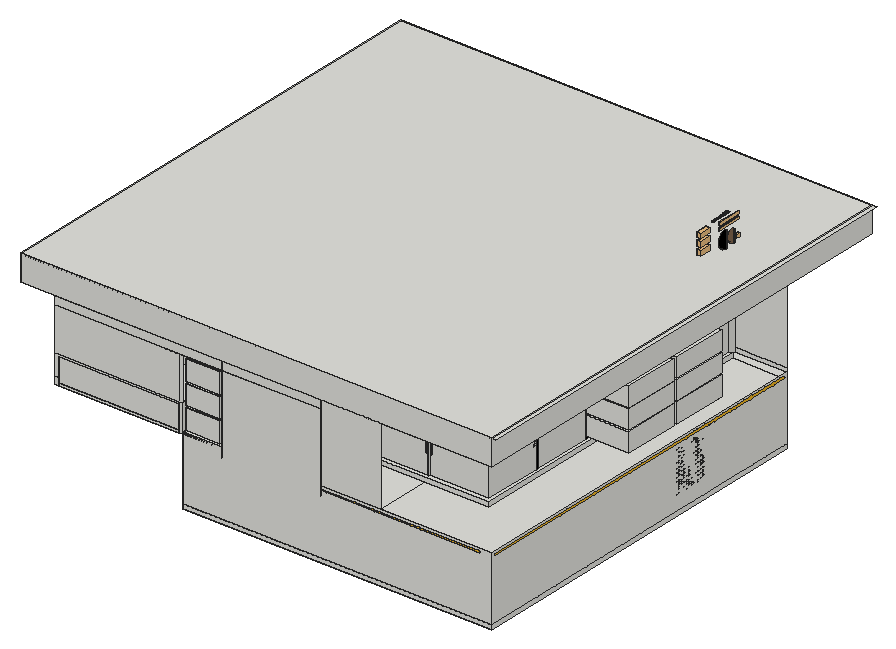
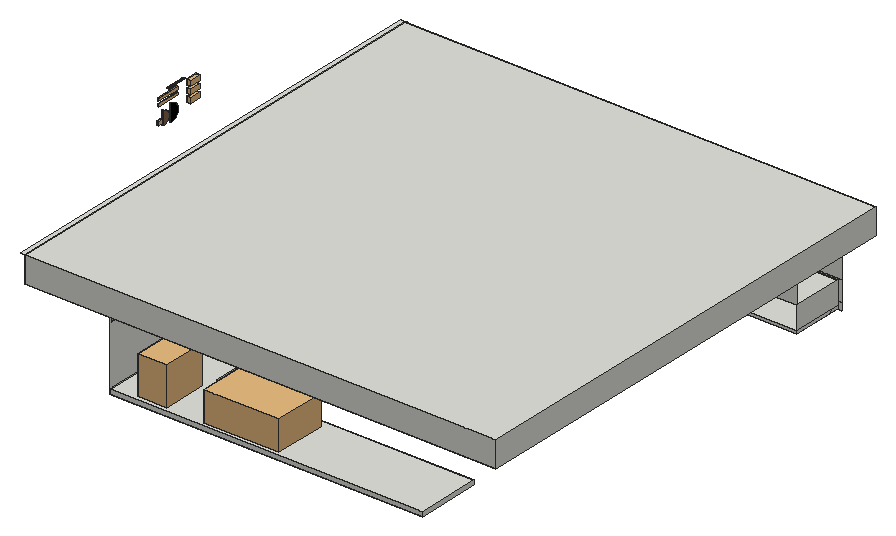
# SketchUp Ruby script. Lengths in inches.
U = 1.inch
M = Sketchup.active_model
def pt(a) = Geom::Point3d.new(a.map { |v| v * U })
def face(e, loops, mat)
  f = e.add_face(loops[0].map { |a| pt(a) })
  loops[1..].each { |l| e.add_face(l.map { |a| pt(a) }).erase! }
  f.material = f.back_material = mat if mat
  f
end
# faces: each face lists its corners as indices into pts; further lists are holes
def faces(e, pts, list, mat = nil) = list.each { |f| face(e, (f[0].is_a?(Array) ? f : [f]).map { |l| l.map { |i| pts[i] } }, mat) }
# xy, xz, yz: faces in a plane at the given z, y or x. An outline is a flat list of corners, or four numbers for a rectangle; further outlines are holes
def ring(l) = l.size == 4 ? [[l[0], l[1]], [l[2], l[1]], [l[2], l[3]], [l[0], l[3]]] : l.each_slice(2).to_a
def flat(e, list, mat, &to3) = list.each { |f| face(e, (f[0].is_a?(Array) ? f : [f]).map { |l| ring(l).map { |u, v| to3.(u, v) } }, mat) }
def xy(e, z, list, mat = nil) = flat(e, list, mat) { |x, y| [x, y, z] }
def xz(e, y, list, mat = nil) = flat(e, list, mat) { |x, z| [x, y, z] }
def yz(e, x, list, mat = nil) = flat(e, list, mat) { |y, z| [x, y, z] }
def lines(e, pts, list) = list.each { |a, b| e.add_line(pt(pts[a]), pt(pts[b])) }
# prism: a flat outline (further loops are holes) pulled along v
def prism(e, loops, v, mat = nil)
  f = face(e, loops, mat); d = Geom::Vector3d.new(v.map { |x| x * U })
  f.pushpull(f.normal.samedirection?(d) ? d.length : -d.length)
end
def box(e, o, s, mat = nil) = prism(e, [[o, [o[0] + s[0], o[1], o[2]], [o[0] + s[0], o[1] + s[1], o[2]], [o[0], o[1] + s[1], o[2]]]], [0, 0, s[2]], mat)
def at(x, y, z, deg = 0) = Geom::Transformation.translation(pt([x, y, z])) * Geom::Transformation.rotation(ORIGIN, Z_AXIS, deg.degrees)
def axes(o, x, y, z) = Geom::Transformation.new([*x, 0, *y, 0, *z, 0, *pt(o).to_a, 1])
def part(name) = M.definitions.add(name)
# library, detail: a bought-in or finely detailed component or shape, given as its bounding box
def library(name, o, s) = part(name).tap { |d| box(d.entities, o, s) }
def detail(e, o, s) = box(e.add_group.entities, o, s)
def put(e, d, t, mat = nil) = e.add_instance(d, t).tap { |i| i.material = mat if mat }
def group(e, t, mat = nil) = e.add_group.tap { |g| g.transformation = t; g.material = mat if mat }.entities
root = M.entities
M.materials.add("Heather_PantShadow").color = [238, 181, 37]
M.materials.add("Polytec Natio Walnut").color = [132, 104, 79]
M.materials.add("[Color M09]").color = [0, 0, 0]
M.materials.add("[Translucent Glass Blue]").color = [100, 149, 237]
M.materials["[Translucent Glass Blue]"].alpha = 0.5
M.materials.add("cnwhc.com_草图联盟_1kmauOsh").color = [54, 52, 52]
M.materials.add("cnwhc.com_草图联盟_C8Y5Xp2O").color = [156, 156, 156]
M.materials["cnwhc.com_草图联盟_C8Y5Xp2O"].alpha = 0.15
M.materials.add("cnwhc.com_草图联盟_IHFcDxe1").color = [138, 151, 59]
M.materials.add("cnwhc.com_草图联盟_KNEfX85g").color = [162, 126, 87]
M.materials.add("cnwhc.com_草图联盟_QJow1Ky4").color = [144, 133, 65]
M.materials.add("cnwhc.com_草图联盟_z6N5x4Hv").color = [237, 222, 58]
c1 = library("Potted plant",[0.24,-1.94,0],[14.49,14.49,6.23])
c2 = library("Plant",[-15.17,-14.95,0],[35.27,31.45,46.14])
c3 = library("Bosch Stove",[0,0,0],[36.22,20.12,1.38])
c4 = library("Group\#260",[0,0,0],[30.82,7.02,10])
c5 = library("Group\#49",[-248.47,-468.28,0.39],[392.05,393.05,278.56])
c6 = library("Food+(14)",[-17.72,-12.23,0],[35.37,24.44,13.82])
c7 = library("Group\#43",[91.875,-459.8125,1.36],[84.84,84.82,167.94])
c8 = library("Group\#47",[175.77,-498.01,1.36],[84.71,84.74,167.94])
c9 = library("Group\#44",[93.63,-458.06,3.28],[81.33,81.31,90.04])
c10 = library("Group\#46",[177.52,-496.26,3.28],[81.21,81.23,127.94])
c11 = library("Group\#50",[-141.57,-278.65,11.2],[96.36,96.33,131.41])
c12 = library("Group\#51",[-62.08,-202.43,11.2],[96.04,96.07,131.41])
c13 = library("Group\#52",[18.13,-280.93,11.2],[96.51,96.54,131.41])
c14 = library("Group\#53",[-213.25,-366.61,11.2],[96.18,96.15,131.41])
c15 = library("Group\#60",[-138.35,-437.94,11.2],[96.49,96.52,131.41])
c16 = library("Group\#54",[-61.03,-358.93,11.2],[96.54,96.51,131.41])
c17 = library("Group\#59",[-225.25,-376.69,19.19],[116.52,116.69,261.73])
c18 = library("Group\#61",[-142.58,-458.38,19.87],[79.66,135.74,256])
c19 = library("Group\#55",[8.05,-292.87,22.71],[116.19,111.01,218.49])
c20 = library("Group\#57",[-143.92,-281.53,22.82],[119.68,105.06,218.38])
c21 = library("Group\#58",[-64.19,-232.55,22.9],[102.65,128.29,224.14])
c22 = library("Group\#56",[-64.85,-368.89,23],[127.95,108.9,222.0625])
c23 = library("Group\#42",[118.34,-437.05,68.8],[33.09,42.97,27.32])
c24 = library("Group\#48",[198.24,-475.92,149.53],[39.78,40.55,40.71])
c25 = library("Group\#45",[114.46,-437.1875,150.05],[39.68,39.57,39.67])
c26 = library("Lg+Water+purifier (1)",[0,2.4,0],[10.83,14.37,19.92])
c27 = library("Chimney",[0,-14.34,0],[33.95,14.34,33.72])
c28 = library("Group\#130",[-198.8,84.74,613.85],[84,84,172.39])
c29 = library("Group\#129",[-105.26,84.74,613.85],[84,84,172.39])
c30 = library("Group\#123",[-15.73,84.74,613.85],[84,84,172.39])
c31 = library("Group\#35",[-453.95,-270.9,-0.08],[243.89,243.63,216.82])
c32 = library("78970097",[-100,-100,0],[200,200,30])
c33 = library("78970100",[-75,-75,0],[150,150,60])
c34 = part("232mm Slimline Handle")
detail(c34.entities,[0,0,0],[9.13,0.47,1.38])
c35 = library("Group\#132",[-374.05,84.21,613.65],[72.44,72.44,111.8])
c36 = library("Group\#131",[-289.4,84.22,613.65],[72.44,72.43,111.8])
c37 = library("Group\#133",[-462.66,84.21,613.65],[72.44,72.44,111.8])
c38 = part("232mm Slimline Handle\#1")
detail(c38.entities,[0,0,0],[9.13,0.47,1.38])
c39 = library("Group\#115",[-254.81,120.48,-0.6],[108.21,108.21,334.5])
c40 = library("Group\#117",[-504.125,120.57,-0.1],[108.2,108.21,338.13])
c41 = library("Group\#116",[-376.9,120.94,-0.1],[107.79,107.8,326.37])
c42 = library("Group\#113",[0.46,121.12,-0.1],[106.94,106.94,338.14])
c43 = library("Group\#114",[-133.01,121.19,-0.1],[106.95,106.95,324.89])
c44 = library("Group77\#2",[-35,-35,0],[70,70,205])
c45 = library("Group76\#2",[-35,-35,0],[70,70,205])
c46 = part("200mm Half Round Handle")
xz(c46.entities,0,[[3.9375,0,3.9375,7.875,3.42,7.84,2.92,7.74,2.43,7.57,1.97,7.35,1.54,7.06,1.15,6.72,0.8125,6.33,0.53,5.91,0.3,5.44,0.13,4.96,0.03,4.45,0,3.9375,0.03,3.42,0.13,2.92,0.3,2.43,0.53,1.97,0.8125,1.54,1.15,1.15,1.54,0.8125,1.97,0.53,2.43,0.3,2.92,0.13,3.42,0.03]],"[Color M09]")
xz(c46.entities,0.12,[[3.82,0.01,3.42,0.03,2.92,0.13,2.43,0.3,1.97,0.53,1.54,0.8125,1.15,1.15,0.8125,1.54,0.53,1.97,0.3,2.43,0.13,2.92,0.03,3.42,0,3.9375,0.03,4.45,0.13,4.96,0.3,5.44,0.53,5.91,0.8125,6.33,1.15,6.72,1.54,7.06,1.97,7.35,2.43,7.57,2.92,7.74,3.42,7.84,3.82,7.87]],"[Color M09]")
xz(c46.entities,0.91,[[3.9375,0,3.82,0.01,3.82,7.87,3.9375,7.875]],"[Color M09]")
yz(c46.entities,3.82,[[0.12,0.01,0.91,7.87]],"[Color M09]")
yz(c46.entities,3.9375,[[0,0,0.91,7.875]],"[Color M09]")
p = [[3.42,0,0.03],[2.92,0,0.13],[2.92,0.12,0.13],[3.42,0.12,0.03],[3.9375,0,0],[3.82,0.12,0.01],
  [3.82,0.91,0.01],[3.9375,0.91,0],[2.43,0,0.3],[2.43,0.12,0.3],[1.97,0,0.53],[1.97,0.12,0.53],
  [1.54,0,0.8125],[1.54,0.12,0.8125],[1.15,0,1.15],[1.15,0.12,1.15],[0.8125,0,1.54],[0.8125,0.12,1.54],
  [0.53,0,1.97],[0.53,0.12,1.97],[0.3,0,2.43],[0.3,0.12,2.43],[0.13,0,2.92],[0.13,0.12,2.92],
  [0.03,0,3.42],[0.03,0.12,3.42],[0,0,3.9375],[0,0.12,3.9375],[0.03,0,4.45],[0.03,0.12,4.45],
  [0.13,0,4.96],[0.13,0.12,4.96],[0.3,0,5.44],[0.3,0.12,5.44],[0.53,0,5.91],[0.53,0.12,5.91],
  [0.8125,0,6.33],[0.8125,0.12,6.33],[1.15,0,6.72],[1.15,0.12,6.72],[1.54,0,7.06],[1.54,0.12,7.06],
  [1.97,0,7.35],[1.97,0.12,7.35],[2.43,0,7.57],[2.43,0.12,7.57],[2.92,0,7.74],[2.92,0.12,7.74],
  [3.42,0,7.84],[3.42,0.12,7.84],[3.9375,0,7.875],[3.9375,0.91,7.875],[3.82,0.91,7.87],[3.82,0.12,7.87]]
faces(c46.entities,p,[[0,1,2,3],[4,0,3,5,6,7],[1,8,9,2],[8,10,11,9],[10,12,13,11],[12,14,15,13],[14,16,17,15],[16,18,19,17],
  [18,20,21,19],[20,22,23,21],[22,24,25,23],[24,26,27,25],[26,28,29,27],[28,30,31,29],[30,32,33,31],[32,34,35,33],
  [34,36,37,35],[36,38,39,37],[38,40,41,39],[40,42,43,41],[42,44,45,43],[44,46,47,45],[46,48,49,47],[48,50,51,52,53,49]],"[Color M09]")
c47 = part("150mm Half Round Handle")
xz(c47.entities,0,[[0,0,0.12,0.01,0.12,5.9,0,5.91]],"Polytec Natio Walnut")
xz(c47.entities,0.79,[[0.12,0.01,0.39,0.03,0.76,0.1,1.13,0.22,1.48,0.4,1.8,0.61,2.09,0.86,2.34,1.16,2.56,1.48,2.73,1.82,2.85,2.1875,2.93,2.57,2.95,2.95,2.93,3.34,2.85,3.72,2.73,4.08,2.56,4.43,2.34,4.75,2.09,5.04,1.8,5.3,1.48,5.51,1.13,5.68,0.76,5.8,0.39,5.88,0.12,5.9]],"Polytec Natio Walnut")
xz(c47.entities,0.91,[[0,0,0,5.91,0.39,5.88,0.76,5.8,1.13,5.68,1.48,5.51,1.8,5.3,2.09,5.04,2.34,4.75,2.56,4.43,2.73,4.08,2.85,3.72,2.93,3.34,2.95,2.95,2.93,2.57,2.85,2.1875,2.73,1.82,2.56,1.48,2.34,1.16,2.09,0.86,1.8,0.61,1.48,0.4,1.13,0.22,0.76,0.1,0.39,0.03]],"Polytec Natio Walnut")
yz(c47.entities,0,[[0,0,0.91,5.91]],"Polytec Natio Walnut")
yz(c47.entities,0.12,[[0,0.01,0.79,5.9]],"Polytec Natio Walnut")
p = [[0,0.91,0],[0.39,0.91,0.03],[0.39,0.79,0.03],[0.12,0.79,0.01],[0.12,0,0.01],[0,0,0],
  [0.76,0.91,0.1],[0.76,0.79,0.1],[1.13,0.91,0.22],[1.13,0.79,0.22],[1.48,0.91,0.4],[1.48,0.79,0.4],
  [1.8,0.91,0.61],[1.8,0.79,0.61],[2.09,0.91,0.86],[2.09,0.79,0.86],[2.34,0.91,1.16],[2.34,0.79,1.16],
  [2.56,0.91,1.48],[2.56,0.79,1.48],[2.73,0.91,1.82],[2.73,0.79,1.82],[2.85,0.91,2.1875],[2.85,0.79,2.1875],
  [2.93,0.91,2.57],[2.93,0.79,2.57],[2.95,0.91,2.95],[2.95,0.79,2.95],[2.93,0.91,3.34],[2.93,0.79,3.34],
  [2.85,0.91,3.72],[2.85,0.79,3.72],[2.73,0.91,4.08],[2.73,0.79,4.08],[2.56,0.91,4.43],[2.56,0.79,4.43],
  [2.34,0.91,4.75],[2.34,0.79,4.75],[2.09,0.91,5.04],[2.09,0.79,5.04],[1.8,0.91,5.3],[1.8,0.79,5.3],
  [1.48,0.91,5.51],[1.48,0.79,5.51],[1.13,0.91,5.68],[1.13,0.79,5.68],[0.76,0.91,5.8],[0.76,0.79,5.8],
  [0.39,0.91,5.88],[0.39,0.79,5.88],[0,0.91,5.91],[0,0,5.91],[0.12,0,5.9],[0.12,0.79,5.9]]
faces(c47.entities,p,[[0,1,2,3,4,5],[1,6,7,2],[6,8,9,7],[8,10,11,9],[10,12,13,11],[12,14,15,13],[14,16,17,15],[16,18,19,17],
  [18,20,21,19],[20,22,23,21],[22,24,25,23],[24,26,27,25],[26,28,29,27],[28,30,31,29],[30,32,33,31],[32,34,35,33],
  [34,36,37,35],[36,38,39,37],[38,40,41,39],[40,42,43,41],[42,44,45,43],[44,46,47,45],[46,48,49,47],[48,50,51,52,53,49]],"Polytec Natio Walnut")
c48 = part("Door Lever\#2")
detail(c48.entities,[0,0,0],[5.43,2.05,2.36])
c49 = part("Door Lever\#3")
detail(c49.entities,[0,0,0],[5.43,2.05,2.36])
c50 = part("Group\#346")
detail(c50.entities,[0,0,0],[11.18,0.75,1.1])
c51 = part("Door Lever\#1")
detail(c51.entities,[0,0,0],[5.43,2.05,2.36])
c52 = part("148mm Black Satin Pull\#1")
prism(c52.entities,[[[5.83,0.12,0.5],[5.83,0.16,0.49],[5.83,0.16,0],[5.83,0.31,0],[5.83,0.31,0.49],[5.83,0.35,0.5],[5.83,0.4,0.54],[5.83,0.44,0.59],[5.83,0.46,0.65],[5.83,0.47,0.71],[5.83,0.46,0.77],[5.83,0.44,0.83],[5.83,0.4,0.875],[5.83,0.35,0.91],[5.83,0.3,0.9375],[5.83,0.24,0.94],[5.83,0.18,0.9375],[5.83,0.12,0.91],[5.83,0.07,0.875],[5.83,0.03,0.83],[5.83,0.01,0.77],[5.83,0,0.71],[5.83,0.01,0.65],[5.83,0.03,0.59],[5.83,0.07,0.54]]],[-5.83,0,0],"[Color M09]")
p = [[5.83,0.16,0.59],[0,0.16,0.59],[5.83,0.31,0.59],[0,0.31,0.59]]
lines(c52.entities,p,[[0,1],[2,3]])
xy(root,40,[[[85,9.1,85,33.1,114.61,33.1,114.61,32.7,115.41,32.7,115.41,33.1,144.61,33.1,144.61,32.7,145.41,32.7,145.41,33.1,174.62,33.1,174.62,32.7,175.42,32.7,175.42,33.1,205.03,33.1,205.03,73.11,205.43,73.11,205.43,75.11,205.03,75.11,205.03,85.125,227.03,85.125,227.03,105.125,205.03,105.125,205.03,111.12,205.23,111.12,205.23,113.12,205.03,113.12,205.03,151.125,83,151.125,83,181.125,227.03,181.125,227.03,179.125,229.03,179.125,229.03,9.1],[84.33,179.58,226.64,180.15]],[114.61,32.7,114.61,33.1,85,33.1,85,35.1,203.03,35.1,203.03,33.1,175.42,33.1,175.42,32.7,174.62,32.7,174.62,33.1,145.41,33.1,145.41,32.7,144.61,32.7,144.61,33.1,115.41,33.1,115.41,32.7],[203.03,33.1,203.03,151.125,205.03,151.125,205.03,113.12,205.23,113.12,205.23,111.12,205.03,111.12,205.03,75.11,205.43,75.11,205.43,73.11,205.03,73.11,205.03,33.1],[113.54,153.125,114.54,153.33],[144.2,153.125,145.2,153.53],
  [174.86,153.125,175.86,153.33],[227.03,179.125,229.03,181.125]])
xy(root,40,[[84.33,179.58,226.64,180.15]],"Heather_PantShadow")
xy(root,42,[[85,9.1,229.03,9.1,229.03,83.125,203.03,83.125,203.03,35.1,85,35.1],[[203.03,83.125,229.03,107.125],[205.03,85.125,227.03,105.125]],[203.03,107.125,229.03,107.125,229.03,181.125,83,181.125,83,151.125,203.03,151.125]])
xy(root,71,[[27,9.1,83,33.1]])
xy(root,72,[[85,9.1,103,33.1],[149.03,9.1,177.03,35.1],[177.03,9.1,177.03,35.1,207.03,35.1,207.03,177.125,229.03,177.125,229.03,9.1],[205.03,177.125,229.03,181.125]])
xy(root,72.3125,[[27,9.1,83,33.1]])
xy(root,73,[[86,9.1,102,33.1]])
xy(root,74,[[149.03,35.1,149.03,37.1,176.73,37.1,176.73,36.9,177.32,36.9,177.32,37.35,205.03,37.35,205.03,64.81,205.43,64.81,205.43,65.41,205.03,65.41,205.03,162.82,205.23,162.82,205.23,163.42,205.03,163.42,205.03,177.125,207.03,177.125,207.03,35.1]])
xy(root,75,[[205.03,94.11,225.03,120.12],[205.03,122.12,225.03,148.12]])
xy(root,82.5,[[[86,9.1,102,33.1],[86.08,9.54,101.83,10.61]]])
xy(root,82.5,[[86.08,9.54,101.83,10.61]],"Heather_PantShadow")
xy(root,83,[[[27,9.1,27,33.1,45.37,33.1,45.37,32.9,45.97,32.9,45.97,33.1,64.03,33.1,64.03,32.9,64.63,32.9,64.63,33.1,83,33.1,83,9.1],[46.34,14.58,57.53,16.08]]])
xy(root,83,[[46.34,14.58,57.53,16.08]],"Heather_PantShadow")
xy(root,83.5,[[86,9.1,102,33.1]])
xy(root,84.03,[[[205.03,94.11,225.03,120.12],[218.98,94.6875,222.04,119.6875]],[[205.03,122.12,225.03,148.12],[218.98,122.6875,222.04,147.6875]]])
xy(root,84.03,[[218.98,94.6875,222.04,119.6875],[218.98,122.6875,222.04,147.6875]],"Heather_PantShadow")
xy(root,84.63,[[205.03,94.11,225.03,120.12],[205.03,122.12,225.03,148.12]])
xy(root,92.5,[[[86,9.1,102,33.1],[86.08,9.54,101.83,10.61]]])
xy(root,92.5,[[86.08,9.54,101.83,10.61]],"Heather_PantShadow")
xy(root,93.37,[[[205.03,94.11,225.03,120.12],[218.98,94.625,222.04,119.625]],[[205.03,122.12,225.03,148.12],[218.98,122.6875,222.04,147.6875]]])
xy(root,93.37,[[218.98,94.625,222.04,119.625],[218.98,122.6875,222.04,147.6875]],"Heather_PantShadow")
xy(root,93.5,[[86,9.1,102,33.1]])
xy(root,93.97,[[205.03,94.11,225.03,120.12],[205.03,122.12,225.03,148.12]])
xy(root,103,[[[86,9.1,102,33.1],[86.08,9.54,101.83,10.61]],[[205.03,94.11,225.03,120.12],[218.98,94.6875,222.04,119.6875]],[[205.03,122.12,225.03,148.12],[218.98,122.6875,222.04,147.6875]]])
xy(root,103,[[86.08,9.54,101.83,10.61],[218.98,94.6875,222.04,119.6875],[218.98,122.6875,222.04,147.6875]],"Heather_PantShadow")
xy(root,104,[[25,9.1,103,9.1,103,33.1,64.63,33.1,64.63,32.9,64.03,32.9,64.03,33.1,45.97,33.1,45.97,32.9,45.37,32.9,45.37,33.1,25,33.1],[176.73,36.9,177.32,37.1],[177.32,37.1,205.03,37.35],[205.03,64.81,205.43,65.41],[205.03,162.82,205.23,163.42]])
xy(root,108,[[149.03,9.1,229.03,9.1,229.03,181.125,205.03,181.125,205.03,37.1,149.03,37.1]])
xy(root,120,[[9,9,229.03,9.1],[229.03,9,231,231]])
xz(root,9.1,[[85,40,229.03,42],[[85,42,85,72,103,72,103,104,149.03,104,149.03,72,229.03,72,229.03,42],[149.79,69.95,223.98,71.02],[85.29,71.06,102.6,71.62]],[25,71,27,74.3125],[27,71,83,72.3125],[83,71,85,84],
  [149.03,72,177.03,108],[27,72.3125,83,83],[86,73,102,82.5],[25,74.3125,25,84,83,84,83,83,27,83,27,74.3125],[86,83.5,102,92.5],
  [25,84,83,104],[83,84,85,104],[86,93.5,102,103],[25,104,149.03,108]])
xz(root,9.1,[[149.79,69.95,223.98,71.02],[85.29,71.06,102.6,71.62]],"Heather_PantShadow")
xz(root,32.9,[[45.37,83,45.97,104],[64.03,83,64.63,104]],"[Color M09]")
xz(root,33.1,[[27,71,83,72.3125],[27,83,45.37,104],[45.97,83,64.03,104],[64.63,83,83,104]])
xz(root,33.1,[[[85,72,103,104],[86,73,102,103]],[86,82.5,102,83.5],[86,92.5,102,93.5]],"[Color M09]")
xz(root,33.1,[[86,73,102,82.5],[86,83.5,102,92.5],[86,93.5,102,103]],"[Translucent Glass Blue]")
xz(root,35.1,[[85,40,203.03,42],[149.03,72,207.03,74]])
xz(root,36.9,[[176.73,74,177.32,104]],"[Color M09]")
xz(root,37.1,[[149.03,74,176.73,104],[149.03,104,205.03,108]])
xz(root,37.35,[[177.32,74,205.03,104]])
xz(root,64.81,[[205.03,74,205.43,104]])
xz(root,65.41,[[205.03,74,205.43,104]])
xz(root,85.125,[[205.03,40,227.03,42]])
xz(root,94.11,[[205.03,75,225.03,84.03],[205.03,84.63,225.03,93.37],[205.03,93.97,225.03,103]])
xz(root,105.125,[[205.03,40,227.03,42]])
xz(root,120.12,[[205.03,75,225.03,84.03],[205.03,84.63,225.03,93.37],[205.03,93.97,225.03,103]])
xz(root,122.12,[[205.03,75,225.03,84.03],[205.03,84.63,225.03,93.37],[205.03,93.97,225.03,103]])
xz(root,148.12,[[205.03,75,225.03,84.03],[205.03,84.63,225.03,93.37],[205.03,93.97,225.03,103]])
xz(root,151.125,[[83,40,203.03,42]])
xz(root,162.82,[[205.03,74,205.23,104]])
xz(root,163.42,[[205.03,74,205.23,104]])
xz(root,177.125,[[205.03,72,207.03,74]])
xz(root,181.125,[[83,40,229.03,42],[205.03,72,229.03,74],[205.03,74,229.03,108]])
yz(root,27,[[9.1,71,13.1,72.3125],[13.1,71,33.1,72.3125],[9.1,72.3125,33.1,83]])
yz(root,45.37,[[32.9,83,33.1,84],[32.9,84,33.1,104]])
yz(root,45.97,[[32.9,83,33.1,84],[32.9,84,33.1,104]])
yz(root,64.03,[[32.9,83,33.1,84],[32.9,84,33.1,104]])
yz(root,64.63,[[32.9,83,33.1,84],[32.9,84,33.1,104]])
yz(root,83,[[151.125,40,181.125,42],[9.1,71,13.1,72.3125],[13.1,71,33.1,72.3125],[9.1,72.3125,33.1,83]])
yz(root,85,[[9.1,40,33.1,42],[33.1,40,35.1,42],[9.1,42,33.1,72],[9.1,72,33.1,84]])
yz(root,86,[[9.1,73,33.1,82.5],[9.1,83.5,33.1,92.5],[9.1,93.5,33.1,103]])
yz(root,102,[[9.1,73,33.1,82.5],[9.1,83.5,33.1,92.5],[9.1,93.5,33.1,103]])
yz(root,103,[[9.1,72,33.1,104]])
yz(root,149.03,[[9.1,72,9.1,104,37.1,104,37.1,74,35.1,74,35.1,72],[9.1,104,37.1,108]])
yz(root,176.73,[[36.9,74,37.1,104]])
yz(root,177.32,[[36.9,74,37.35,104]])
yz(root,203.03,[[35.1,40,151.125,42]])
yz(root,205.03,[[85.125,40,105.125,42],[177.125,72,177.125,104,37.1,104,37.1,108,181.125,108,181.125,72],[37.35,74,64.81,104],[65.41,74,93.11,104],[149.12,74,162.82,104],
  [163.42,74,177.125,104]])
yz(root,205.03,[[[93.11,74,149.12,104],[94.11,75,148.12,103]],[120.12,75,122.12,103],[94.11,84.03,120.12,84.63],[122.12,84.03,148.12,84.63],[94.11,93.37,120.12,93.97],
  [122.12,93.37,148.12,93.97]],"[Color M09]")
yz(root,205.03,[[94.11,75,120.12,84.03],[122.12,75,148.12,84.03],[94.11,84.63,120.12,93.37],[122.12,84.63,148.12,93.37],[94.11,93.97,120.12,103],
  [122.12,93.97,148.12,103]],"[Translucent Glass Blue]")
yz(root,205.23,[[162.82,74,163.42,104]],"[Color M09]")
yz(root,205.43,[[64.81,74,65.41,104]],"[Color M09]")
yz(root,207.03,[[35.1,72,177.125,74]])
yz(root,225.03,[[94.11,75,120.12,84.03],[122.12,75,148.12,84.03],[94.11,84.63,120.12,93.37],[122.12,84.63,148.12,93.37],[94.11,93.97,120.12,103],
  [122.12,93.97,148.12,103]])
yz(root,227.03,[[85.125,40,105.125,42]])
yz(root,229.03,[[9.1,40,181.125,42],[[9.1,42,181.125,72],[10.07,69.75,180.01,71.3125]]])
yz(root,229.03,[[10.07,69.75,180.01,71.3125]],"Heather_PantShadow")
p = [[83,9.1,84],[83,33.1,84]]
lines(root,p,[[0,1]])
detail(root,[102.6,33.4375,74.6875],[0.31,0.9,5.98])
detail(root,[102.6,33.4375,85.1875],[0.31,0.9,5.98])
detail(root,[102.6,33.4375,95.375],[0.31,0.9,5.98])
put(root,c1,axes([211.3,17.54,42],[0.63381,0,0],[0,0.73527,0],[0,0,0.80856]))
put(root,c2,axes([210.14,168.18,42],[0.385,0,0],[0,0.6505,0],[0,0,0.385]))
put(root,c3,at(150.25,32.67,42,-180))
put(root,c2,axes([93.02,23.21,42],[0.385,0,0],[0,0.6505,0],[0,0,0.385]))
put(root,c4,at(211.05,64.06,42,-90))
put(root,c5,axes([188.29,35.32,41.98],[0.04248,0,0],[0,0.04248,0],[0,0,0.04248]),"cnwhc.com_草图联盟_1kmauOsh")
put(root,c6,at(169.28,167.06,42))
put(root,c7,axes([188.29,35.32,41.98],[0.04248,0,0],[0,0.04248,0],[0,0,0.04248]),"cnwhc.com_草图联盟_C8Y5Xp2O")
put(root,c8,axes([188.29,35.32,41.98],[0.04248,0,0],[0,0.04248,0],[0,0,0.04248]),"cnwhc.com_草图联盟_C8Y5Xp2O")
put(root,c9,axes([188.29,35.32,41.98],[0.04248,0,0],[0,0.04248,0],[0,0,0.04248]),"cnwhc.com_草图联盟_QJow1Ky4")
put(root,c10,axes([188.29,35.32,41.98],[0.04248,0,0],[0,0.04248,0],[0,0,0.04248]),"cnwhc.com_草图联盟_z6N5x4Hv")
put(root,c11,axes([188.29,35.32,41.98],[0.04248,0,0],[0,0.04248,0],[0,0,0.04248]),"cnwhc.com_草图联盟_C8Y5Xp2O")
put(root,c12,axes([188.29,35.32,41.98],[0.04248,0,0],[0,0.04248,0],[0,0,0.04248]),"cnwhc.com_草图联盟_C8Y5Xp2O")
put(root,c13,axes([188.29,35.32,41.98],[0.04248,0,0],[0,0.04248,0],[0,0,0.04248]),"cnwhc.com_草图联盟_C8Y5Xp2O")
put(root,c14,axes([188.29,35.32,41.98],[0.04248,0,0],[0,0.04248,0],[0,0,0.04248]),"cnwhc.com_草图联盟_C8Y5Xp2O")
put(root,c15,axes([188.29,35.32,41.98],[0.04248,0,0],[0,0.04248,0],[0,0,0.04248]),"cnwhc.com_草图联盟_C8Y5Xp2O")
put(root,c16,axes([188.29,35.32,41.98],[0.04248,0,0],[0,0.04248,0],[0,0,0.04248]),"cnwhc.com_草图联盟_C8Y5Xp2O")
put(root,c17,axes([188.29,35.32,41.98],[0.04248,0,0],[0,0.04248,0],[0,0,0.04248]))
put(root,c18,axes([188.29,35.32,41.98],[0.04248,0,0],[0,0.04248,0],[0,0,0.04248]))
put(root,c19,axes([188.29,35.32,41.98],[0.04248,0,0],[0,0.04248,0],[0,0,0.04248]),"cnwhc.com_草图联盟_1kmauOsh")
put(root,c20,axes([188.29,35.32,41.98],[0.04248,0,0],[0,0.04248,0],[0,0,0.04248]),"cnwhc.com_草图联盟_1kmauOsh")
put(root,c21,axes([188.29,35.32,41.98],[0.04248,0,0],[0,0.04248,0],[0,0,0.04248]),"cnwhc.com_草图联盟_1kmauOsh")
put(root,c22,axes([188.29,35.32,41.98],[0.04248,0,0],[0,0.04248,0],[0,0,0.04248]),"cnwhc.com_草图联盟_1kmauOsh")
put(root,c23,axes([188.29,35.32,41.98],[0.04248,0,0],[0,0.04248,0],[0,0,0.04248]),"cnwhc.com_草图联盟_IHFcDxe1")
put(root,c24,axes([188.29,35.32,41.98],[0.04248,0,0],[0,0.04248,0],[0,0,0.04248]),"cnwhc.com_草图联盟_KNEfX85g")
put(root,c25,axes([188.29,35.32,41.98],[0.04248,0,0],[0,0.04248,0],[0,0,0.04248]),"cnwhc.com_草图联盟_KNEfX85g")
put(root,c26,axes([229.03,135.41,49.03],[-0.89,0,0],[0,-1.10645,0],[0,0,0.9879]))
put(root,c27,axes([149.03,9.27,67.53],[-1.3558,0,0],[0,-1,0],[0,0,1.2]))
put(root,c1,axes([49.59,23.85,72.3125],[0.51114,0,0],[0,0.44837,0],[0,0,0.52185]))
put(root,c28,axes([90.82,32.63,44.15],[-0.047,0,0],[0,-0.047,0],[0,0,0.047]))
put(root,c29,axes([90.82,32.63,44.15],[-0.047,0,0],[0,-0.047,0],[0,0,0.047]))
put(root,c30,axes([90.82,32.63,44.15],[-0.047,0,0],[0,-0.047,0],[0,0,0.047]))
put(root,c31,axes([227.02,142.13,75],[0.04453,0,0],[0,0.04494,0],[0,0,0.03706]))
put(root,c32,axes([214.75,106.03,75],[0,0.04661,0],[0.04661,0,0],[0,0,0.04661]))
put(root,c32,axes([214.79,106.12,75.93],[0.03296,0.03296,0],[0.03296,-0.03296,0],[0,0,0.04661]))
put(root,c32,axes([214.7,106.03,76.86],[0.03296,0.03296,0],[0.03296,-0.03296,0],[0,0,0.04661]))
put(root,c33,axes([214.75,105.5625,77.8],[-0.03296,0.03296,0],[0.03296,0.03296,0],[0,0,0.04661]))
put(root,c34,axes([177.86,37.35,82.9],[0,0,1],[1,0,0],[0,1,0]),"[Color M09]")
put(root,c34,axes([175.65,37.35,82.9],[0,0,1],[1,0,0],[0,1,0]),"[Color M09]")
put(root,c35,axes([78.73,34.2,55.48],[-0.04567,0,0],[0,-0.04567,0],[0,0,0.04567]))
put(root,c36,axes([78.73,34.2,55.48],[-0.04567,0,0],[0,-0.04567,0],[0,0,0.04567]))
put(root,c37,axes([78.73,34.2,55.48],[-0.04567,0,0],[0,-0.04567,0],[0,0,0.04567]))
put(root,c34,axes([205.03,63.84,83.54],[0,0,1],[0,1,0],[-1,0,0]),"[Color M09]")
put(root,c34,axes([205.03,65.84,83.54],[0,0,1],[0,1,0],[-1,0,0]),"[Color M09]")
put(root,c33,axes([214.27,105.64,84.63],[-0.03296,0.03296,0],[0.03296,0.03296,0],[0,0,0.04661]))
put(root,c31,axes([227.02,142.13,84.64],[0.04453,0,0],[0,0.04494,0],[0,0,0.03706]))
put(root,c38,axes([204.79,120.23,85.39],[0,0,0.8265],[0,0.8265,0],[-0.8265,0,0]),"[Color M09]")
put(root,c38,axes([204.79,121.35,85.39],[0,0,0.8265],[0,0.8265,0],[-0.8265,0,0]),"[Color M09]")
put(root,c33,axes([214.18,105.73,86.96],[0,0.04661,0],[0.04661,0,0],[0,0,0.04661]))
put(root,c33,axes([214.23,105.68,89.29],[0.03296,0.03296,0],[0.03296,-0.03296,0],[0,0,0.04661]))
put(root,c34,axes([65.63,33.1,89.7],[0,0,1],[1,0,0],[0,1,0]),"[Color M09]")
put(root,c34,axes([62.38,33.1,89.7],[0,0,1],[1,0,0],[0,1,0]),"[Color M09]")
put(root,c34,axes([43.76,33.1,89.7],[0,0,1],[1,0,0],[0,1,0]),"[Color M09]")
put(root,c39,axes([98.11,24.22,93.5],[0.0198,0,0],[0,0.0198,0],[0,0,0.0198]))
put(root,c40,axes([98.11,24.22,93.5],[0.0198,0,0],[0,0.0198,0],[0,0,0.0198]))
put(root,c41,axes([98.11,24.22,93.5],[0.0198,0,0],[0,0.0198,0],[0,0,0.0198]))
put(root,c42,axes([98.11,24.22,93.5],[0.0198,0,0],[0,0.0198,0],[0,0,0.0198]))
put(root,c43,axes([98.11,24.22,93.5],[0.0198,0,0],[0,0.0198,0],[0,0,0.0198]))
put(root,c31,axes([227.02,142.13,93.97],[0.04453,0,0],[0,0.04494,0],[0,0,0.03706]))
put(root,c44,axes([211.41,106.5,93.97],[0,0.04661,0],[0.04661,0,0],[0,0,0.04661]))
put(root,c45,axes([211.41,103,93.97],[0.04661,0,0],[0,-0.04661,0],[0,0,0.04661]))
g1 = group(root,at(9,9.1,120))
xy(g1,-12,[[[0,0,220.03,221.9],[24,24,196.03,197.9]],[28,28,192.03,193.9]])
xy(g1,-12,[[[24,24,196.03,197.9],[28,28,192.03,193.9]]],"cnwhc.com_草图联盟_z6N5x4Hv")
xy(g1,0,[[0,0,220.03,221.9]])
xz(g1,0,[[0,-12,220.03,0]])
xz(g1,221.9,[[0,-12,220.03,0]])
yz(g1,0,[[0,-12,221.9,0]])
yz(g1,220.03,[[0,-12,221.9,0]])
put(root,c46,axes([228.12,142.57,146.55],[0,1,0],[1,0,0],[0,0,-1]))
put(root,c47,axes([229.03,150.9,145.32],[0,-1,0],[-1,0,0],[0,0,-1]))
g2 = group(root,at(227.84,153.93,140.69,-90))
detail(g2,[0,0,0],[1.58,1.18,1.58])
put(root,c48,at(226.98,136.45,142.5,-90))
put(root,c49,at(226.98,136.45,146.11,-90))
put(root,c50,at(228.28,153.4,148.16,-90))
put(root,c51,at(226.98,136.45,149.71,-90))
g3 = group(root,at(228.28,153.4,150.42,-90))
detail(g3,[0,0,0],[11.18,0.75,1.1])
g4 = group(root,at(227.61,148.03,153.28,-90))
prism(g4,[[[2.36,0.48,0.13],[2.36,0.5,0.18],[2.36,1.42,0.18],[2.36,1.42,0.33],[2.36,0.5,0.33],[2.36,0.48,0.38],[2.36,0.4375,0.4375],[2.36,0.38,0.48],[2.36,0.32,0.5],[2.36,0.26,0.51],[2.36,0.19,0.5],[2.36,0.13,0.48],[2.36,0.07,0.4375],[2.36,0.03,0.38],[2.36,0.01,0.32],[2.36,0,0.26],[2.36,0.01,0.19],[2.36,0.03,0.13],[2.36,0.07,0.07],[2.36,0.13,0.03],[2.36,0.19,0.01],[2.36,0.26,0],[2.36,0.32,0.01],[2.36,0.38,0.03],[2.36,0.4375,0.07]]],[-2.36,0,0])
put(root,c52,axes([229.03,144.36,153.3],[0,-1,0],[0,0,1],[-1,0,0]))
